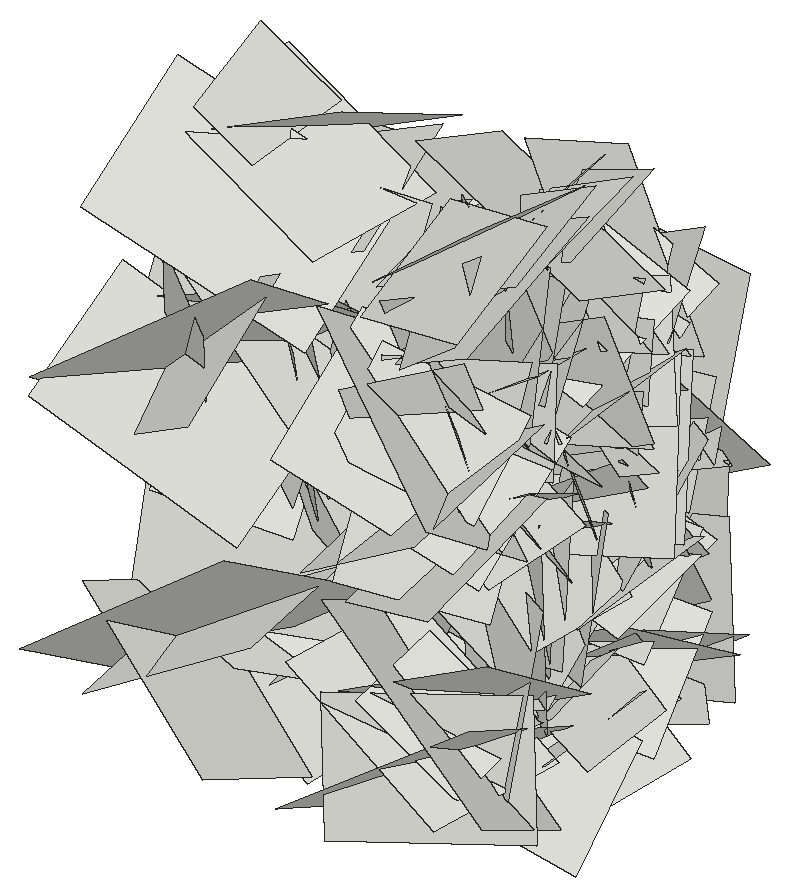
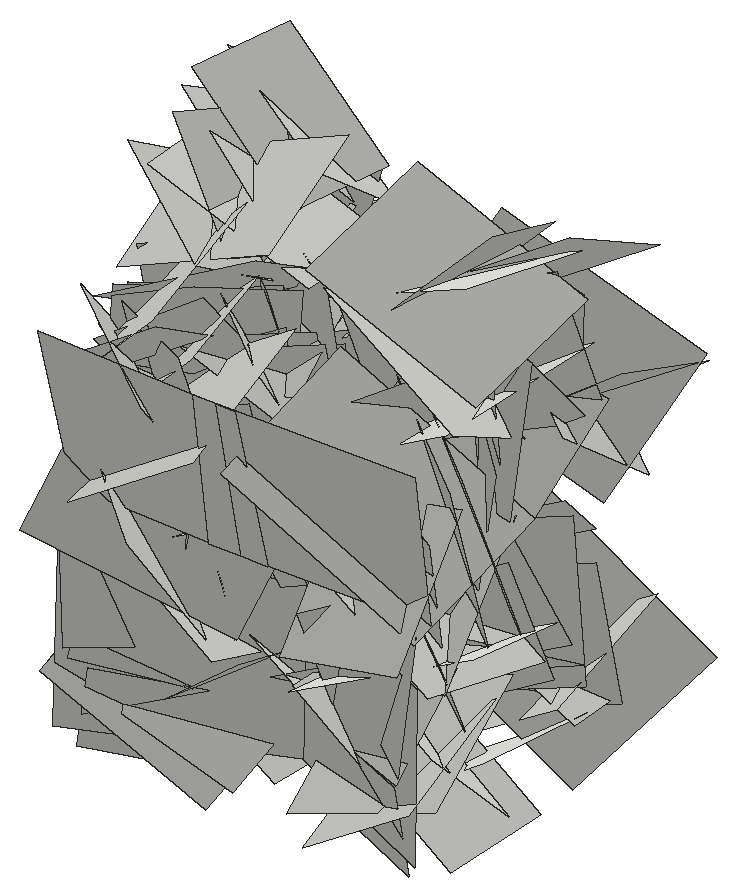
# SketchUp Ruby script. Lengths in inches.
U = 1.inch
M = Sketchup.active_model
def pt(a) = Geom::Point3d.new(a.map { |v| v * U })
def face(e, loops, mat)
  f = e.add_face(loops[0].map { |a| pt(a) })
  loops[1..].each { |l| e.add_face(l.map { |a| pt(a) }).erase! }
  f.material = f.back_material = mat if mat
  f
end
# faces: each face lists its corners as indices into pts; further lists are holes
def faces(e, pts, list, mat = nil) = list.each { |f| face(e, (f[0].is_a?(Array) ? f : [f]).map { |l| l.map { |i| pts[i] } }, mat) }
# xy, xz, yz: faces in a plane at the given z, y or x. An outline is a flat list of corners, or four numbers for a rectangle; further outlines are holes
def ring(l) = l.size == 4 ? [[l[0], l[1]], [l[2], l[1]], [l[2], l[3]], [l[0], l[3]]] : l.each_slice(2).to_a
def flat(e, list, mat, &to3) = list.each { |f| face(e, (f[0].is_a?(Array) ? f : [f]).map { |l| ring(l).map { |u, v| to3.(u, v) } }, mat) }
def xy(e, z, list, mat = nil) = flat(e, list, mat) { |x, y| [x, y, z] }
def xz(e, y, list, mat = nil) = flat(e, list, mat) { |x, z| [x, y, z] }
def yz(e, x, list, mat = nil) = flat(e, list, mat) { |y, z| [x, y, z] }
def lines(e, pts, list) = list.each { |a, b| e.add_line(pt(pts[a]), pt(pts[b])) }
# prism: a flat outline (further loops are holes) pulled along v
def prism(e, loops, v, mat = nil)
  f = face(e, loops, mat); d = Geom::Vector3d.new(v.map { |x| x * U })
  f.pushpull(f.normal.samedirection?(d) ? d.length : -d.length)
end
def box(e, o, s, mat = nil) = prism(e, [[o, [o[0] + s[0], o[1], o[2]], [o[0] + s[0], o[1] + s[1], o[2]], [o[0], o[1] + s[1], o[2]]]], [0, 0, s[2]], mat)
def at(x, y, z, deg = 0) = Geom::Transformation.translation(pt([x, y, z])) * Geom::Transformation.rotation(ORIGIN, Z_AXIS, deg.degrees)
def axes(o, x, y, z) = Geom::Transformation.new([*x, 0, *y, 0, *z, 0, *pt(o).to_a, 1])
def part(name) = M.definitions.add(name)
# library, detail: a bought-in or finely detailed component or shape, given as its bounding box
def library(name, o, s) = part(name).tap { |d| box(d.entities, o, s) }
def detail(e, o, s) = box(e.add_group.entities, o, s)
def put(e, d, t, mat = nil) = e.add_instance(d, t).tap { |i| i.material = mat if mat }
def group(e, t, mat = nil) = e.add_group.tap { |g| g.transformation = t; g.material = mat if mat }.entities
root = M.entities
c1 = part("Component\#6")
p = [[0.01,0,0],[0,3.24,4.54],[4.32,3.24,4.54],[4.33,0,0]]
faces(c1.entities,p,[[0,1,2,3]])
put(root,c1,axes([18.5,211.4,20.36],[0.11841,0.02386,0.67628],[-0.07272,0.6823,-0.01274],[-0.7136,-0.06557,0.11352]))
put(root,c1,axes([14.53,209.77,25.57],[-0.04769,1.02209,-0.46416],[-0.05126,-0.46587,-1.02116],[1.18879,0.02092,-0.06265]))
put(root,c1,axes([14.53,212.41,27.7],[0.11035,-0.46639,-0.85158],[-0.0233,-0.85737,0.46687],[1.02892,0.03061,0.1019]))
put(root,c1,axes([18.5,210.37,37.54],[0.0852,-0.7988,-0.26142],[0.21653,-0.23617,0.78446],[-0.8642,-0.13792,0.17078]))
put(root,c1,axes([18.5,207.84,29.22],[0.13906,-0.51177,-0.49755],[-0.00544,-0.50655,0.51967],[-0.75658,-0.09042,-0.09518]))
put(root,c1,axes([14.53,211.63,27.44],[0.13698,0.50835,-0.7639],[0.02564,-0.77306,-0.51036],[0.97231,-0.05123,0.12108]))
put(root,c1,axes([14.53,212.85,24.81],[-0.10314,-0.72888,-0.73382],[0.20394,-0.73695,0.70648],[1.07722,0.06973,-0.20401]))
put(root,c1,axes([14.53,211.43,33.78],[-0.23599,-0.36182,-1.29322],[-0.09706,-1.30373,0.38052],[1.42014,-0.14923,-0.18889]))
put(root,c1,axes([14.53,199.54,32.72],[-0.14681,1.15124,0.44909],[-0.05729,0.44582,-1.15954],[1.30862,0.14867,-0.00039]))
put(root,c1,axes([14.53,206.07,20.81],[-0.31441,-1.20333,0.63493],[-0.01893,0.65323,1.22967],[1.44208,-0.25378,0.15457]))
put(root,c1,axes([14.53,208.01,36.375],[-0.10923,0.38133,-1.06486],[0.05778,-1.06635,-0.38714],[1.19755,0.08623,-0.07845]))
put(root,c1,axes([14.53,212.99,32.26],[0.05541,-0.21084,-0.92918],[0.15034,-0.91849,0.21639],[0.99872,0.14996,0.01898]))
put(root,c1,axes([14.53,205.46,33.43],[0.14097,0.63084,0.7943],[-0.06243,0.80455,-0.62912],[1.07339,-0.03606,-0.14091]))
put(root,c1,axes([14.53,207.91,30.98],[-0.03881,-0.77727,0.6188],[0.26695,0.59174,0.75817],[1.01873,-0.18467,-0.1751]))
put(root,c1,axes([18.5,206,31.6],[0.1462,-0.08624,0.716],[0.07336,0.72719,0.07426],[-0.76092,0.05354,0.14472]))
put(root,c1,axes([18.5,210.56,30.82],[0.08988,0.23539,0.56706],[-0.00516,0.57268,-0.23699],[-0.65079,0.02797,0.0802]))
put(root,c1,axes([14.53,206.55,33.15],[0.00164,-0.95203,-0.71322],[-0.09471,-0.7113,0.94927],[1.25737,-0.05234,0.07244]))
put(root,c1,axes([14.53,206.8125,26.89],[-0.15204,1.11982,0.24611],[0.19339,0.26716,-1.10927],[1.19986,0.09884,0.20998]))
put(root,c1,axes([14.53,211.99,33.59],[-0.13241,-0.25962,-1.28668],[-0.09489,-1.2878,0.26854],[1.38813,-0.1128,-0.10438]))
put(root,c1,axes([14.53,206.95,24.98],[0.09414,0.39654,1.07266],[-0.12922,1.07305,-0.38659],[1.20532,0.08407,-0.12522]))
put(root,c1,axes([18.5,202.49,32.61],[0.11645,-0.17214,0.59947],[0.01233,0.60916,0.17278],[-0.661,-0.01896,0.10883]))
put(root,c1,axes([14.53,205.38,23.16],[0.04798,1.09948,0.05597],[0.01409,0.05547,-1.10036],[1.16688,-0.04588,0.01099]))
put(root,c1,axes([14.53,210.75,36.02],[-0.14272,-1.0645,0.43866],[0.22696,0.41079,1.0626],[1.19913,-0.20445,-0.14891]))
put(root,c1,axes([14.53,208.81,31.45],[-0.04602,0.84125,-1.04893],[-0.18208,-1.04435,-0.83047],[1.4136,-0.10713,-0.14111]))
put(root,c1,axes([14.53,213.59,29.33],[0.10669,0.07311,-1.12569],[-0.06812,-1.12796,-0.079],[1.19381,-0.0709,0.09609]))
put(root,c1,axes([14.53,201.95,25.76],[0.02109,1.10253,-0.4508],[-0.04504,-0.44992,-1.10225],[1.2618,-0.03449,-0.03181]))
put(root,c1,axes([14.53,213.06,27.02],[-0.109,-1.16412,-0.17966],[0.1638,-0.19212,1.15639],[1.23778,-0.07709,-0.16885]))
put(root,c1,axes([14.53,201.85,37.73],[-0.10519,1.13817,0.58904],[-0.00109,0.59073,-1.14161],[1.35845,0.08861,0.0447]))
put(root,c1,axes([14.53,204.59,30.02],[-0.04301,-1.09683,0.72238],[-0.12053,0.72294,1.0913],[1.38692,0.02882,0.11724]))
put(root,c1,axes([14.53,209.74,33.23],[0.15201,0.07034,-1.21602],[-0.20156,-1.20811,-0.09231],[1.2753,-0.19933,0.13035]))
put(root,c1,axes([14.53,208.94,26.04],[-0.1299,1.02121,-0.60997],[0.25035,-0.5801,-1.01865],[1.23578,0.22487,0.14225]))
put(root,c1,axes([14.53,213.71,29.11],[-0.07729,-1.24842,0.49404],[-0.03127,0.49613,1.24937],[1.42283,-0.05691,0.0543]))
put(root,c1,axes([14.53,211.375,32.78],[-0.08242,0.8278,-0.94283],[0.12426,-0.93571,-0.83122],[1.32412,0.13934,0.01932]))
put(root,c1,axes([14.53,211.85,35.53],[0.11979,-0.95717,-0.48165],[0.13908,-0.46832,0.96146],[1.12727,0.15949,-0.06744]))
put(root,c1,axes([14.53,203.71,22.72],[-0.0324,0.32539,1.27516],[0.00551,1.27553,-0.32536],[1.39498,0.00251,0.0309]))
put(root,c1,axes([14.53,205.99,22.98],[0.14358,-1.11124,-0.06865],[0.09474,-0.05808,1.11649],[1.17635,0.14031,-0.08154]))
put(root,c1,axes([14.53,205.63,39.17],[0.17317,1.06099,0.10432],[0.22006,0.07185,-1.05594],[1.10844,-0.18002,0.19334]))
put(root,c1,axes([14.53,205.46,24.09],[0.08024,0.04196,1.34674],[-0.06239,1.34768,-0.03868],[1.42687,0.05657,-0.07742]))
put(root,c1,axes([14.53,204.65,33.57],[0.11682,0.36237,1.1463],[0.15256,1.13885,-0.37385],[1.26518,-0.17079,-0.06076]))
put(root,c1,axes([14.53,211.92,20.51],[0.20622,-1.25394,-0.15944],[-0.06822,-0.17093,1.26581],[1.33814,0.18453,0.0891]))
put(root,c1,axes([14.53,213.57,27.56],[-0.01798,0.03957,-1.39555],[0.22262,-1.3797,-0.04168],[1.46303,0.21042,-0.01081]))
put(root,c1,axes([14.53,205.51,24.88],[0.13882,1.11155,0.63897],[0.19603,0.6192,-1.11507],[1.34484,-0.205,0.09658]))
put(root,c1,axes([14.19,214.11,35.21],[0.07772,-0.27644,-1.33377],[0.91911,-1.02064,0.2592],[1.11351,0.86175,-0.12086]))
put(root,c1,axes([14.53,205.05,35.75],[0.23328,1.34713,-0.22992],[0.05022,-0.24027,-1.36238],[1.44774,-0.20874,0.08431]))
put(root,c1,axes([14.53,206.12,25.83],[0.28838,0.48251,1.20317],[0.13396,1.21365,-0.51529],[1.36755,-0.22063,-0.20324]))
put(root,c1,axes([28.31,206.12,25.83],[-0.28838,0.48251,1.20317],[-0.13396,1.21365,-0.51529],[-1.36755,-0.22063,-0.20324]))
put(root,c1,axes([28.31,205.05,35.75],[-0.23328,1.34713,-0.22992],[-0.05022,-0.24027,-1.36238],[-1.44774,-0.20874,0.08431]))
put(root,c1,axes([28.65,214.11,35.21],[-0.07772,-0.27644,-1.33377],[-0.91911,-1.02064,0.2592],[-1.11351,0.86175,-0.12086]))
put(root,c1,axes([28.31,205.51,24.88],[-0.13882,1.11155,0.63897],[-0.19603,0.6192,-1.11507],[-1.34484,-0.205,0.09658]))
put(root,c1,axes([28.31,213.57,27.56],[0.01798,0.03957,-1.39555],[-0.22262,-1.3797,-0.04168],[-1.46303,0.21042,-0.01081]))
put(root,c1,axes([28.31,211.92,20.51],[-0.20622,-1.25394,-0.15944],[0.06822,-0.17093,1.26581],[-1.33814,0.18453,0.0891]))
put(root,c1,axes([28.31,204.65,33.57],[-0.11682,0.36237,1.1463],[-0.15256,1.13885,-0.37385],[-1.26518,-0.17079,-0.06076]))
put(root,c1,axes([28.31,205.46,24.09],[-0.08024,0.04196,1.34674],[0.06239,1.34768,-0.03868],[-1.42687,0.05657,-0.07742]))
put(root,c1,axes([28.31,205.63,39.17],[-0.17317,1.06099,0.10432],[-0.22006,0.07185,-1.05594],[-1.10844,-0.18002,0.19334]))
put(root,c1,axes([28.31,205.99,22.98],[-0.14358,-1.11124,-0.06865],[-0.09474,-0.05808,1.11649],[-1.17635,0.14031,-0.08154]))
put(root,c1,axes([28.31,203.71,22.72],[0.0324,0.32539,1.27516],[-0.00551,1.27553,-0.32536],[-1.39498,0.00251,0.0309]))
put(root,c1,axes([28.31,211.85,35.53],[-0.11979,-0.95717,-0.48165],[-0.13908,-0.46832,0.96146],[-1.12727,0.15949,-0.06744]))
put(root,c1,axes([28.31,211.375,32.78],[0.08242,0.8278,-0.94283],[-0.12426,-0.93571,-0.83122],[-1.32412,0.13934,0.01932]))
put(root,c1,axes([28.31,213.71,29.11],[0.07729,-1.24842,0.49404],[0.03127,0.49613,1.24937],[-1.42283,-0.05691,0.0543]))
put(root,c1,axes([28.31,208.94,26.04],[0.1299,1.02121,-0.60997],[-0.25035,-0.5801,-1.01865],[-1.23578,0.22487,0.14225]))
put(root,c1,axes([28.31,209.74,33.23],[-0.15201,0.07034,-1.21602],[0.20156,-1.20811,-0.09231],[-1.2753,-0.19933,0.13035]))
put(root,c1,axes([28.31,204.59,30.02],[0.04301,-1.09683,0.72238],[0.12053,0.72294,1.0913],[-1.38692,0.02882,0.11724]))
put(root,c1,axes([28.31,201.85,37.73],[0.10519,1.13817,0.58904],[0.00109,0.59073,-1.14161],[-1.35845,0.08861,0.0447]))
put(root,c1,axes([28.31,213.06,27.02],[0.109,-1.16412,-0.17966],[-0.1638,-0.19212,1.15639],[-1.23778,-0.07709,-0.16885]))
put(root,c1,axes([28.31,201.95,25.76],[-0.02109,1.10253,-0.4508],[0.04504,-0.44992,-1.10225],[-1.2618,-0.03449,-0.03181]))
put(root,c1,axes([28.31,213.59,29.33],[-0.10669,0.07311,-1.12569],[0.06812,-1.12796,-0.079],[-1.19381,-0.0709,0.09609]))
put(root,c1,axes([28.31,208.81,31.45],[0.04602,0.84125,-1.04893],[0.18208,-1.04435,-0.83047],[-1.4136,-0.10713,-0.14111]))
put(root,c1,axes([28.31,210.75,36.02],[0.14272,-1.0645,0.43866],[-0.22696,0.41079,1.0626],[-1.19913,-0.20445,-0.14891]))
put(root,c1,axes([28.31,205.38,23.16],[-0.04798,1.09948,0.05597],[-0.01409,0.05547,-1.10036],[-1.16688,-0.04588,0.01099]))
put(root,c1,axes([24.34,202.49,32.61],[-0.11645,-0.17214,0.59947],[-0.01233,0.60916,0.17278],[0.661,-0.01896,0.10883]))
put(root,c1,axes([28.31,206.95,24.98],[-0.09414,0.39654,1.07266],[0.12922,1.07305,-0.38659],[-1.20532,0.08407,-0.12522]))
put(root,c1,axes([28.31,211.99,33.59],[0.13241,-0.25962,-1.28668],[0.09489,-1.2878,0.26854],[-1.38813,-0.1128,-0.10438]))
put(root,c1,axes([28.31,206.8125,26.89],[0.15204,1.11982,0.24611],[-0.19339,0.26716,-1.10927],[-1.19986,0.09884,0.20998]))
put(root,c1,axes([28.31,206.55,33.15],[-0.00164,-0.95203,-0.71322],[0.09471,-0.7113,0.94927],[-1.25737,-0.05234,0.07244]))
put(root,c1,axes([24.34,210.56,30.82],[-0.08988,0.23539,0.56706],[0.00516,0.57268,-0.23699],[0.65079,0.02797,0.0802]))
put(root,c1,axes([24.34,206,31.6],[-0.1462,-0.08624,0.716],[-0.07336,0.72719,0.07426],[0.76092,0.05354,0.14472]))
put(root,c1,axes([28.31,207.91,30.98],[0.03881,-0.77727,0.6188],[-0.26695,0.59174,0.75817],[-1.01873,-0.18467,-0.1751]))
put(root,c1,axes([28.31,205.46,33.43],[-0.14097,0.63084,0.7943],[0.06243,0.80455,-0.62912],[-1.07339,-0.03606,-0.14091]))
put(root,c1,axes([28.31,212.99,32.26],[-0.05541,-0.21084,-0.92918],[-0.15034,-0.91849,0.21639],[-0.99872,0.14996,0.01898]))
put(root,c1,axes([28.31,208.01,36.375],[0.10923,0.38133,-1.06486],[-0.05778,-1.06635,-0.38714],[-1.19755,0.08623,-0.07845]))
put(root,c1,axes([28.31,206.07,20.81],[0.31441,-1.20333,0.63493],[0.01893,0.65323,1.22967],[-1.44208,-0.25378,0.15457]))
put(root,c1,axes([28.31,199.54,32.72],[0.14681,1.15124,0.44909],[0.05729,0.44582,-1.15954],[-1.30862,0.14867,-0.00039]))
put(root,c1,axes([28.31,211.43,33.78],[0.23599,-0.36182,-1.29322],[0.09706,-1.30373,0.38052],[-1.42014,-0.14923,-0.18889]))
put(root,c1,axes([28.31,212.85,24.81],[0.10314,-0.72888,-0.73382],[-0.20394,-0.73695,0.70648],[-1.07722,0.06973,-0.20401]))
put(root,c1,axes([28.31,211.63,27.44],[-0.13698,0.50835,-0.7639],[-0.02564,-0.77306,-0.51036],[-0.97231,-0.05123,0.12108]))
put(root,c1,axes([24.34,207.84,29.22],[-0.13906,-0.51177,-0.49755],[0.00544,-0.50655,0.51967],[0.75658,-0.09042,-0.09518]))
put(root,c1,axes([24.34,210.37,37.54],[-0.0852,-0.7988,-0.26142],[-0.21653,-0.23617,0.78446],[0.8642,-0.13792,0.17078]))
put(root,c1,axes([28.31,212.41,27.7],[-0.11035,-0.46639,-0.85158],[0.0233,-0.85737,0.46687],[-1.02892,0.03061,0.1019]))
put(root,c1,axes([28.31,209.77,25.57],[0.04769,1.02209,-0.46416],[0.05126,-0.46587,-1.02116],[-1.18879,0.02092,-0.06265]))
put(root,c1,axes([24.34,211.4,20.36],[-0.11841,0.02386,0.67628],[0.07272,0.6823,-0.01274],[0.7136,-0.06557,0.11352]))
put(root,c1,axes([24.34,208.95,27.68],[-0.1117,0.11156,-0.75397],[-0.06454,-0.75994,-0.10393],[0.80532,-0.04543,-0.11291]))
put(root,c1,axes([24.34,203.96,20.97],[0.02025,-0.24988,0.58047],[-0.03388,0.57961,0.25056],[0.66903,0.03691,-0.00488]))
put(root,c1,axes([24.34,202.42,34.22],[-0.03507,0.56649,-0.26791],[0.06705,-0.26389,-0.56581],[0.66085,0.05684,0.04319]))
put(root,c1,axes([28.31,211.47,22.62],[0.20513,-1.22241,0.07319],[0.04122,0.08019,1.23659],[-1.29742,-0.19072,0.05085]))
put(root,c1,axes([28.31,206.36,33.23],[0.09168,1.1059,0.20164],[0.04784,0.19866,-1.1089],[-1.19063,0.09314,-0.02903]))
put(root,c1,axes([28.31,205.67,24.52],[-0.15369,0.87531,0.08009],[0.01982,0.08422,-0.88666],[-0.9315,-0.14262,-0.03208]))
put(root,c1,axes([28.31,207.21,30.03],[0.00943,-1.01637,-0.0193],[0.00822,-0.01923,1.01638],[-1.07752,-0.00904,0.00758]))
put(root,c1,axes([24.34,204.95,35.05],[0.03568,0.1968,-0.61743],[-0.04358,-0.61637,-0.1987],[0.68554,-0.04943,0.01951]))
put(root,c1,axes([24.34,212.36,26.625],[-0.06935,-0.64087,-0.11796],[0.11905,-0.12787,0.63241],[0.68039,-0.04294,-0.12268]))
put(root,c1,axes([24.34,206.625,39.5],[-0.00312,0.09172,-0.66161],[0.00201,-0.66161,-0.09173],[0.70801,0.00228,-0.00265]))
put(root,c1,axes([24.34,204.22,36.67],[0.08595,0.41822,-0.43473],[-0.01861,-0.43682,-0.42351],[0.63917,-0.06896,0.04613]))
put(root,c1,axes([24.34,202.23,33.91],[0.02493,0.60398,0.49928],[-0.17768,0.49182,-0.58706],[0.81142,0.08914,-0.14389]))
put(root,c1,axes([24.34,200.85,29.625],[-0.04324,0.39016,0.69087],[-0.10275,0.68414,-0.39209],[0.83473,0.10443,-0.01247]))
put(root,c1,axes([24.34,212.78,35.18],[-0.06835,-0.19577,-0.64021],[0.13077,-0.63563,0.18195],[0.69749,0.09999,-0.09685]))
put(root,c1,axes([24.34,211.1,35.2],[0.07899,0.5337,0.27791],[0.02897,0.27674,-0.53878],[0.63716,-0.07875,-0.00996]))
put(root,c1,axes([28.31,202.75,27.49],[0.17368,0.85862,-0.51485],[-0.1903,-0.48804,-0.87105],[-1.04401,0.2318,0.07312]))
put(root,c1,axes([24.34,206.77,29.69],[0.13468,0.0618,0.68245],[-0.14259,0.68282,-0.03679],[0.71222,0.12502,-0.13642]))
put(root,c1,axes([28.31,204.74,34.65],[-0.08046,-0.48471,-0.63269],[-0.12911,-0.62103,0.49039],[-0.83492,0.14274,-0.01486]))
put(root,c1,axes([28.31,210.61,30.96],[-0.02538,-1.03384,0.49264],[0.2847,0.47394,1.00764],[-1.18007,0.13657,0.23251]))
put(root,c1,axes([28.31,212.48,33.12],[-0.02538,-1.03384,0.49264],[0.2847,0.47394,1.00764],[-1.18007,0.13657,0.23251]))
put(root,c1,axes([28.31,201.41,38.375],[0.12316,0.77538,0.57304],[-0.12545,0.58429,-0.76661],[-1.01427,0.02189,0.1644]))
put(root,c1,axes([24.34,207.11,31.75],[-0.23783,0.22127,0.93353],[-0.03566,0.95632,-0.23476],[1.01634,0.08533,0.21022]))
put(root,c1,axes([28.31,210.23,35.31],[-0.06568,0.00099,-0.81141],[-0.08224,-0.81005,0.00494],[-0.85616,0.07773,0.06177]))
put(root,c1,axes([24.34,204.33,34.72],[-0.02793,-0.28222,0.66343],[0.05268,0.66158,0.28341],[0.7624,-0.05605,0.00473]))
put(root,c1,axes([24.34,209.27,26.93],[0.01951,-0.6006,0.29742],[0.06663,0.29777,0.59742],[0.70729,-0.01148,-0.06448]))
put(root,c1,axes([28.31,205.35,34.65],[-0.12302,0.37909,0.72016],[0.00858,0.72795,-0.38188],[-0.86263,-0.04682,-0.1065]))
put(root,c1,axes([28.31,204.65,32.19],[-0.14144,0.68446,-0.34907],[-0.03425,-0.35898,-0.69154],[-0.81371,-0.10387,0.08978]))
put(root,c1,axes([24.34,205,37.54],[0.1597,-0.46751,-0.41946],[-0.05532,-0.43919,0.47075],[0.66349,0.07592,0.14021]))
put(root,c1,axes([28.31,204.82,25.65],[0.12938,-0.11687,-1.00907],[-0.02351,-1.01639,0.11504],[-1.07651,0.00815,-0.12379]))
put(root,c1,axes([24.34,211.91,37.97],[-0.10192,-0.72839,-0.40458],[-0.00784,-0.4065,0.73361],[0.88316,-0.08767,-0.04018]))
put(root,c1,axes([24.34,207.4,37.82],[-0.14382,-0.92009,0.02073],[-0.06912,0.03051,0.92748],[0.97309,-0.13382,0.06894]))
put(root,c1,axes([28.31,206.58,28.49],[-0.01093,-0.51913,0.63451],[-0.10311,0.63085,0.51456],[-0.86287,-0.06881,-0.06953]))
put(root,c1,axes([24.34,201.89,25.36],[0.12511,0.60489,0.30184],[-0.04372,0.31228,-0.60968],[0.71524,-0.08672,-0.09007]))
put(root,c1,axes([24.34,209.37,33.75],[-0.00852,0.3462,-0.76666],[-0.09329,-0.76284,-0.34355],[0.88678,-0.07692,-0.04351]))
put(root,c1,axes([28.31,210.92,34.25],[-0.13403,0.53039,0.57824],[0.04314,0.58935,-0.53168],[-0.83061,-0.05497,-0.12092]))
put(root,c1,axes([24.34,209.14,33.82],[0.16184,0.36707,0.52708],[-0.01835,0.54392,-0.37378],[0.68059,-0.07262,-0.13541]))
put(root,c1,axes([28.31,204.07,39.0625],[0.02986,0.79051,0.40956],[-0.00815,0.40997,-0.79076],[-0.94369,0.02147,0.01979]))
put(root,c1,axes([24.34,207.43,34.16],[0.11276,0.04323,0.70746],[-0.03845,0.71477,-0.03823],[0.75032,0.03013,-0.10828]))
put(root,c1,axes([28.31,200.125,30.08],[0.25415,0.9144,0.59243],[0.00684,0.60541,-0.93704],[-1.1549,0.20481,0.12483]))
put(root,c1,axes([28.31,209.72,22.08],[0.18138,-0.91546,-0.54155],[0.07402,-0.53767,0.93095],[-1.12504,-0.18297,-0.02606]))
put(root,c1,axes([28.31,208.86,27.22],[0.22907,0.58895,0.94038],[0.09031,0.94642,-0.61231],[-1.17269,0.18793,0.13653]))
put(root,c1,axes([28.31,209.27,26.87],[-0.02942,-0.98917,0.00062],[0.2303,-0.00549,0.9654],[-1.02292,0.02721,0.21733]))
put(root,c1,axes([24.34,202.89,32.22],[-0.0211,0.0618,0.84202],[-0.01452,0.84212,-0.06213],[0.89482,0.01512,0.01885]))
put(root,c1,axes([28.31,210.17,27.25],[-0.0389,-0.19659,0.74237],[-0.03773,0.74285,0.19496],[-0.81316,-0.02506,-0.04456]))
